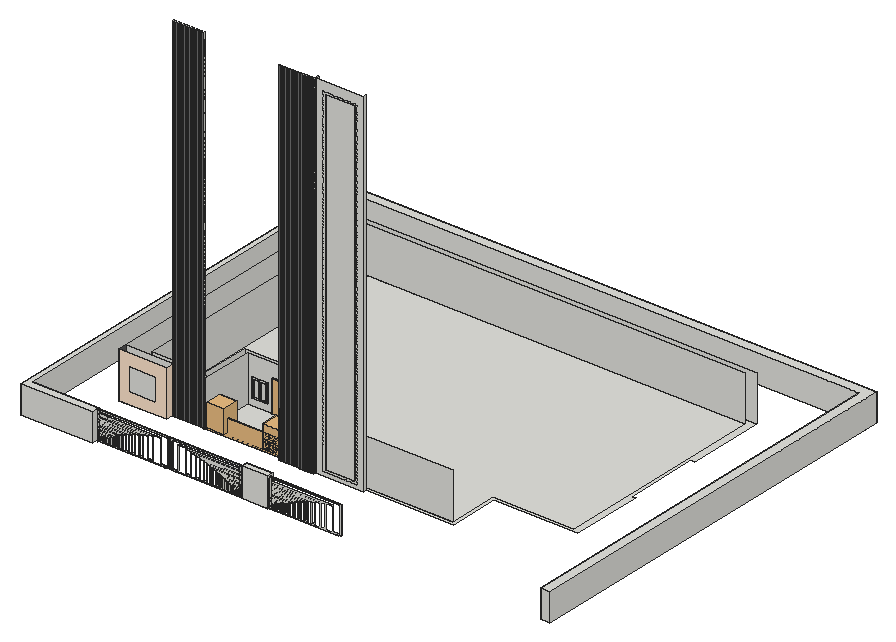
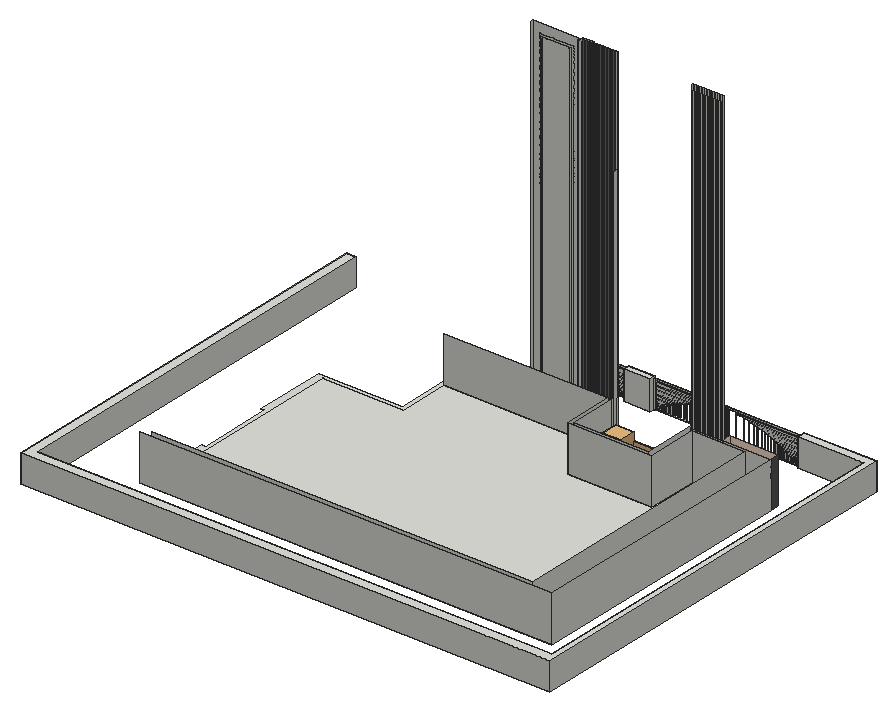
# SketchUp Ruby script. Lengths in inches.
U = 1.inch
M = Sketchup.active_model
def pt(a) = Geom::Point3d.new(a.map { |v| v * U })
def face(e, loops, mat)
  f = e.add_face(loops[0].map { |a| pt(a) })
  loops[1..].each { |l| e.add_face(l.map { |a| pt(a) }).erase! }
  f.material = f.back_material = mat if mat
  f
end
# faces: each face lists its corners as indices into pts; further lists are holes
def faces(e, pts, list, mat = nil) = list.each { |f| face(e, (f[0].is_a?(Array) ? f : [f]).map { |l| l.map { |i| pts[i] } }, mat) }
# xy, xz, yz: faces in a plane at the given z, y or x. An outline is a flat list of corners, or four numbers for a rectangle; further outlines are holes
def ring(l) = l.size == 4 ? [[l[0], l[1]], [l[2], l[1]], [l[2], l[3]], [l[0], l[3]]] : l.each_slice(2).to_a
def flat(e, list, mat, &to3) = list.each { |f| face(e, (f[0].is_a?(Array) ? f : [f]).map { |l| ring(l).map { |u, v| to3.(u, v) } }, mat) }
def xy(e, z, list, mat = nil) = flat(e, list, mat) { |x, y| [x, y, z] }
def xz(e, y, list, mat = nil) = flat(e, list, mat) { |x, z| [x, y, z] }
def yz(e, x, list, mat = nil) = flat(e, list, mat) { |y, z| [x, y, z] }
def lines(e, pts, list) = list.each { |a, b| e.add_line(pt(pts[a]), pt(pts[b])) }
# prism: a flat outline (further loops are holes) pulled along v
def prism(e, loops, v, mat = nil)
  f = face(e, loops, mat); d = Geom::Vector3d.new(v.map { |x| x * U })
  f.pushpull(f.normal.samedirection?(d) ? d.length : -d.length)
end
def box(e, o, s, mat = nil) = prism(e, [[o, [o[0] + s[0], o[1], o[2]], [o[0] + s[0], o[1] + s[1], o[2]], [o[0], o[1] + s[1], o[2]]]], [0, 0, s[2]], mat)
def at(x, y, z, deg = 0) = Geom::Transformation.translation(pt([x, y, z])) * Geom::Transformation.rotation(ORIGIN, Z_AXIS, deg.degrees)
def axes(o, x, y, z) = Geom::Transformation.new([*x, 0, *y, 0, *z, 0, *pt(o).to_a, 1])
def part(name) = M.definitions.add(name)
# library, detail: a bought-in or finely detailed component or shape, given as its bounding box
def library(name, o, s) = part(name).tap { |d| box(d.entities, o, s) }
def detail(e, o, s) = box(e.add_group.entities, o, s)
def put(e, d, t, mat = nil) = e.add_instance(d, t).tap { |i| i.material = mat if mat }
def group(e, t, mat = nil) = e.add_group.tap { |g| g.transformation = t; g.material = mat if mat }.entities
root = M.entities
M.materials.add("[Color C01]").color = [255, 229, 204]
M.materials.add("[Color M05]").color = [114, 114, 114]
M.materials.add("[Color M06]").color = [86, 86, 86]
c1 = part("Glass Door - Open Shower")
box(c1.entities,[0,0,0.95],[40,1.5,72])
c2 = library("Glass balustrade section",[0,0,0],[60.75,3.875,44.35])
c3 = library("KentiaPalm",[-22.86,-14.31,0],[47.49,43.96,59.125])
c4 = library("porta 4",[0.2,-5.42,1.33],[46.55,4.72,83.21])
c5 = part("Window")
xy(c5.entities,31.72,[[-0.78,88.6,2.72,128.1]])
xy(c5.entities,34.95,[[-0.78,91.53,0.84,106.59],[0.84,91.53,1.05,97.58],[1.05,91.53,1.42,106.59],[1.42,91.53,2.72,106.59],[0.84,97.58,1.05,98.18],
  [0.84,98.18,1.05,106.59]])
xy(c5.entities,35.27,[[-0.78,110.09,0.97,125.14],[1.05,110.09,2.72,125.14]])
xy(c5.entities,58.35,[[2.72,108.74,3.8,109.74]])
xy(c5.entities,77.8125,[[-0.78,110.09,2.72,125.14],[0.97,110.09,1.05,125.14]])
xy(c5.entities,77.93,[[-0.78,91.53,0.84,106.59],[1.05,91.53,1.42,106.59],[1.42,91.53,2.72,106.59]])
xy(c5.entities,80.72,[[-0.78,88.6,2.72,128.1]])
xz(c5.entities,88.6,[[-0.78,31.72,2.72,80.72]])
xz(c5.entities,91.53,[[-0.78,34.95,0.84,77.93],[1.05,34.95,1.42,77.93],[1.42,34.95,2.72,77.93]])
xz(c5.entities,106.59,[[-0.78,34.95,0.84,77.93],[0.84,34.95,1.05,77.93],[0.84,34.95,2.72,77.93]])
xz(c5.entities,108.74,[[3.8,54.35,4.22,54.6,4.22,59.47,2.72,59.97,2.72,58.35,3.8,58.35]])
xz(c5.entities,109.74,[[3.8,54.35,3.8,58.35,2.72,58.35,2.72,59.97,4.22,59.47,4.22,54.6]])
xz(c5.entities,110.09,[[-0.78,35.27,0.97,77.8125],[1.05,35.27,2.72,77.8125]])
xz(c5.entities,125.14,[[-0.78,35.27,0.97,77.8125],[0.97,35.27,1.05,80.72],[1.05,35.27,2.72,77.8125]])
xz(c5.entities,128.1,[[-0.78,31.72,2.72,80.72]])
yz(c5.entities,-0.78,[[[88.6,31.72,128.1,80.72],[91.53,34.95,106.59,77.93],[110.09,35.27,125.14,77.8125]]])
yz(c5.entities,0.84,[[91.53,34.95,106.59,77.93]])
yz(c5.entities,0.97,[[110.09,35.27,125.14,77.8125]])
yz(c5.entities,1.05,[[91.53,34.95,106.59,77.93],[110.09,35.27,125.14,77.8125]])
yz(c5.entities,1.42,[[91.53,34.95,106.59,77.93]])
yz(c5.entities,2.72,[[[88.6,31.72,108.35,80.72],[91.53,34.95,106.59,77.93]],[[108.35,31.72,128.1,80.72],[110.09,35.27,125.14,77.8125],[108.74,58.35,109.74,59.97]]])
yz(c5.entities,3.8,[[108.74,54.35,109.74,58.35]])
yz(c5.entities,4.22,[[108.74,54.6,109.74,59.47]])
p = [[4.22,108.74,54.6],[3.8,108.74,54.35],[3.8,109.74,54.35],[4.22,109.74,54.6],[2.72,109.74,59.97],[2.72,108.74,59.97],
  [4.22,108.74,59.47],[4.22,109.74,59.47],[-0.78,86.4,89.94],[-0.78,86.44,89.94],[15.22,130.69,89.94],[15.22,130.65,89.94],
  [-0.78,86.44,28.19],[-0.78,86.4,28.19],[7.72,130.69,89.94],[7.72,130.65,89.94]]
faces(c5.entities,p,[[0,1,2,3],[4,5,6,7]])
lines(c5.entities,p,[[8,9],[10,11],[12,13],[14,15]])
box(root,[569.26,11.31,0],[68.62,15.69,75.8125])
prism(root,[[[0,1064.875,0],[1383.3125,1064.875,0],[1383.3125,0,0],[1358.82,0,0],[1358.82,1038.875,0],[15.91,1038.875,0],[15.91,21.72,0],[188.09,21.72,0],[188.09,0,0],[0,0,0]]],[0,0,72.6875])
xy(root,0,[[528.5625,182.3125,534.875,184.75],[535.75,182.3125,542.0625,184.75],[542.5,182.3125,548.8125,184.75],[549.375,182.3125,555.6875,184.75],[556.1875,182.3125,562.5,184.75],
  [563.1875,182.3125,569.5,184.75],[570.1875,182.3125,576.5,184.75],[577,182.3125,583.3125,184.75],[584.75,182.3125,591.0625,184.75],[592,182.3125,598.3125,184.75],
  [599.375,182.3125,605.6875,184.75],[606.75,182.3125,613.07,184.75],[614.13,182.3125,620.44,184.75],[[528.67,184.75,620.44,184.75,620.44,195.5625,622.95,195.5625,622.95,187.0625,747.02,187.0625,747.02,195.5625,974.8125,195.5625,974.8125,325.5625,1196,325.5625,1196,513.49,1186.5,513.49,1186.5,706.47,1196,706.47,1196,908.0625,119.8125,908.0625,119.8125,195.5625,327.85,195.5625,327.85,189.875,333.1,189.875,333.1,325.5625,528.67,325.5625],[180.5,204.5625,180.5,894.25,1177.5,894.25,1177.5,334.5625,965.8125,334.5625,965.8125,204.5625,537.67,204.5625,537.67,334.5625,318.85,334.5625,318.85,204.5625]],[244.96,193.5625,325.71,195.5625],
  [333.1,195.5625,528.67,325.5625],[180.5,204.5625,318.85,204.5625,318.85,334.5625,537.67,334.5625,537.67,204.5625,965.8125,204.5625,965.8125,334.5625,1177.5,334.5625,1177.5,894.25,180.5,894.25]])
xy(root,0,[[245.08,191.125,251.39,193.5625],[251.83,191.125,258.14,193.5625],[258.52,191.125,264.83,193.5625],[265.14,191.125,271.46,193.5625],[271.89,191.125,278.21,193.5625],
  [278.64,191.125,284.96,193.5625],[285.46,191.125,291.77,193.5625],[292.21,191.125,298.52,193.5625],[299.02,191.125,305.33,193.5625],[305.83,191.125,312.14,193.5625],
  [312.71,191.125,319.02,193.5625],[319.39,191.125,325.71,193.5625]],"[Color M05]")
xy(root,0,[[119.8125,172.4375,244.96,195.5625]],"[Color M06]")
xy(root,0.49,[[193.54,13.81,370.76,14.31],[385.35,13.81,562.58,14.31],[643.44,13.81,820.67,14.31]])
xy(root,0.7,[[187.97,14.12,191.63,15.56],[372.66,14.12,376.32,15.56],[379.79,14.12,383.45,15.56],[564.48,14.12,568.14,15.56],[637.88,14.12,641.54,15.56]])
xy(root,3.2,[[197.6875,13.81,203.4375,14.31],[206.84,13.81,212.06,14.31],[216.11,13.81,221.45,14.31],[226.23,13.81,231.97,14.31],[237.375,13.81,243.66,14.31],
  [249.79,13.81,256.71,14.31],[263.81,13.81,271.47,14.31],[279.92,13.81,288.49,14.31],[298.9,13.81,308.95,14.31],[321.26,13.81,335.28,14.31],
  [354.73,13.81,366.2,14.31],[366.2,13.81,370.76,14.31],[385.35,13.81,389.91,14.31],[389.91,13.81,401.38,14.31],[420.83,13.81,434.85,14.31],
  [447.17,13.81,457.21,14.31],[467.62,13.81,476.19,14.31],[484.64,13.81,492.31,14.31],[499.4,13.81,506.32,14.31],[512.45,13.81,518.74,14.31],
  [524.14,13.81,529.88,14.31],[534.66,13.81,540,14.31],[544.05,13.81,549.28,14.31],[552.68,13.81,558.43,14.31],[647.59,13.81,653.34,14.31],
  [656.74,13.81,661.97,14.31],[666.01,13.81,671.36,14.31],[676.14,13.81,681.88,14.31],[687.28,13.81,693.57,14.31],[699.7,13.81,706.61,14.31],
  [713.71,13.81,721.38,14.31],[729.83,13.81,738.4,14.31],[748.81,13.81,758.85,14.31]])
xy(root,3.7,[[475.4,13.73,468.41,13.8,468.41,14.31,475.4,14.31],[730.62,13.73,737.61,13.8,737.61,14.31,730.62,14.31],[299.6875,13.93,308.16,14.02,308.16,14.31,299.6875,14.31],[456.42,13.93,447.95,14.02,447.95,14.31,456.42,14.31],[749.6,13.93,758.07,14.02,758.07,14.31,749.6,14.31],
  [322.05,14.17,334.49,14.31,322.05,14.31],[434.07,14.17,421.62,14.31,434.07,14.31]])
xy(root,5.63,[[196.38,13.81,200.95,14.31],[555.16,13.81,559.73,14.31],[646.29,13.81,650.86,14.31]])
xy(root,6.62,[[193.54,13.81,194.89,14.31],[194.89,13.81,196.01,14.31],[196.01,13.81,203.4375,14.31],[552.68,13.81,560.1,14.31],[560.1,13.81,561.22,14.31],
  [561.22,13.81,562.58,14.31],[643.44,13.81,644.8,14.31],[644.8,13.81,645.92,14.31],[645.92,13.81,653.34,14.31]])
xy(root,9.32,[[193.54,13.81,199.38,14.31],[199.38,13.81,200.99,14.31],[200.99,13.81,206.84,14.31],[549.28,13.81,555.12,14.31],[555.12,13.81,556.73,14.31],
  [556.73,13.81,562.58,14.31],[643.44,13.81,649.29,14.31],[649.29,13.81,650.9,14.31],[650.9,13.81,656.74,14.31]])
xy(root,12.74,[[193.54,13.81,204.26,14.31],[204.26,13.81,212.06,14.31],[544.05,13.81,551.85,14.31],[551.85,13.81,562.58,14.31],[643.44,13.81,654.17,14.31],
  [654.17,13.81,661.97,14.31]])
xy(root,15.44,[[193.54,13.81,209.89,14.31],[209.89,13.81,216.11,14.31],[540,13.81,546.22,14.31],[546.22,13.81,562.58,14.31],[643.44,13.81,659.79,14.31],
  [659.79,13.81,666.01,14.31]])
xy(root,17.65,[[647.73,187.0625,723.37,190.9375]])
xy(root,18.86,[[193.54,13.81,213.58,14.31],[213.58,13.81,221.45,14.31],[534.66,13.81,542.53,14.31],[542.53,13.81,562.58,14.31],[643.44,13.81,663.48,14.31],
  [663.48,13.81,671.36,14.31]])
xy(root,21.57,[[193.54,13.81,219.5625,14.31],[219.5625,13.81,226.23,14.31],[529.88,13.81,536.55,14.31],[536.55,13.81,562.58,14.31],[643.44,13.81,669.47,14.31],
  [669.47,13.81,676.14,14.31]])
xy(root,24.98,[[193.54,13.81,223.73,14.31],[223.73,13.81,231.97,14.31],[524.14,13.81,532.38,14.31],[532.38,13.81,562.58,14.31],[643.44,13.81,673.64,14.31],
  [673.64,13.81,681.88,14.31]])
xz(root,14.12,[[187.97,0.7,187.97,73.2,376.32,73.2,376.32,0.7,372.66,0.7,372.66,70.9,191.63,70.9,191.63,0.7],[379.79,0.7,383.45,0.7,383.45,70.9,564.48,70.9,564.48,0.7,568.14,0.7,568.14,73.2,379.79,73.2],[637.88,0.7,637.88,73.2,826.23,73.2,826.23,0.7,822.57,0.7,822.57,70.9,641.54,70.9,641.54,0.7]])
xz(root,14.31,[[[192.75,0,192.75,3.7,196.01,6.12,202.65,6.12,199.38,3.7,202.65,3.7,202.65,6.12,192.75,6.12,192.75,9.82,207.625,9.82,207.625,3.7,211.27,3.7,211.27,12.24,192.75,12.24,192.75,15.9375,216.9,15.9375,216.9,3.7,220.67,3.7,220.67,18.36,192.75,18.36,192.75,22.06,227.02,22.06,227.02,3.7,231.18,3.7,231.18,24.48,192.75,24.48,192.75,28.18,238.16,28.18,238.16,3.7,242.875,3.7,242.875,30.61,192.75,30.61,192.75,34.3,250.58,34.3,250.58,3.7,255.92,3.7,255.92,36.73,192.75,36.73,192.75,40.42,264.59,40.42,264.59,3.7,270.68,3.7,270.68,42.85,192.75,42.85,192.75,46.54,280.71,46.54,280.71,3.7,287.71,3.7,287.71,48.97,192.75,48.97,192.75,52.67,299.6875,52.67,299.6875,3.7,308.16,3.7,308.16,55.09,192.75,55.09,192.75,58.79,322.05,58.79,322.05,3.7,334.49,3.7,334.49,61.21,192.75,61.21,192.75,64.91,355.52,64.91,355.52,3.7,371.55,3.7,371.55,0],[193.54,0.49,370.76,0.49,370.76,3.2,354.73,3.2,354.73,64.41,193.54,64.41,193.54,61.71,335.28,61.71,335.28,3.2,321.26,3.2,321.26,58.29,193.54,58.29,193.54,55.59,308.95,55.59,308.95,3.2,298.9,3.2,298.9,52.17,193.54,52.17,193.54,49.46,288.49,49.46,288.49,3.2,279.92,3.2,279.92,46.05,193.54,46.05,193.54,43.34,271.47,43.34,271.47,3.2,263.81,3.2,263.81,39.93,193.54,39.93,193.54,37.22,256.71,37.22,256.71,3.2,249.79,3.2,249.79,33.81,193.54,33.81,193.54,31.1,243.66,31.1,243.66,3.2,237.375,3.2,237.375,27.6875,193.54,27.6875,193.54,24.98,231.97,24.98,231.97,3.2,226.23,3.2,226.23,21.57,193.54,21.57,193.54,18.86,221.45,18.86,221.45,3.2,216.11,3.2,216.11,15.44,193.54,15.44,193.54,12.74,212.06,12.74,212.06,3.2,206.84,3.2,206.84,9.32,193.54,9.32,193.54,6.62,203.4375,6.62,203.4375,3.2,197.6875,3.2,200.95,5.63,196.38,5.63,193.54,3.52]],[[384.5625,0,563.36,0,563.36,3.7,560.1,6.12,553.46,6.12,556.73,3.7,553.46,3.7,553.46,6.12,563.36,6.12,563.36,9.82,548.49,9.82,548.49,3.7,544.84,3.7,544.84,12.24,563.36,12.24,563.36,15.9375,539.22,15.9375,539.22,3.7,535.45,3.7,535.45,18.36,563.36,18.36,563.36,22.06,529.09,22.06,529.09,3.7,524.93,3.7,524.93,24.48,563.36,24.48,563.36,28.18,517.95,28.18,517.95,3.7,513.24,3.7,513.24,30.61,563.36,30.61,563.36,34.3,505.53,34.3,505.53,3.7,500.19,3.7,500.19,36.73,563.36,36.73,563.36,40.42,491.52,40.42,491.52,3.7,485.43,3.7,485.43,42.85,563.36,42.85,563.36,46.54,475.4,46.54,475.4,3.7,468.41,3.7,468.41,48.97,563.36,48.97,563.36,52.67,456.42,52.67,456.42,3.7,447.95,3.7,447.95,55.09,563.36,55.09,563.36,58.79,434.07,58.79,434.07,3.7,421.62,3.7,421.62,61.21,563.36,61.21,563.36,64.91,400.59,64.91,400.59,3.7,384.5625,3.7],[385.35,0.49,385.35,3.2,401.38,3.2,401.38,64.41,562.58,64.41,562.58,61.71,420.83,61.71,420.83,3.2,434.85,3.2,434.85,58.29,562.58,58.29,562.58,55.59,447.17,55.59,447.17,3.2,457.21,3.2,457.21,52.17,562.58,52.17,562.58,49.46,467.62,49.46,467.62,3.2,476.19,3.2,476.19,46.05,562.58,46.05,562.58,43.34,484.64,43.34,484.64,3.2,492.31,3.2,492.31,39.93,562.58,39.93,562.58,37.22,499.4,37.22,499.4,3.2,506.32,3.2,506.32,33.81,562.58,33.81,562.58,31.1,512.45,31.1,512.45,3.2,518.74,3.2,518.74,27.6875,562.58,27.6875,562.58,24.98,524.14,24.98,524.14,3.2,529.88,3.2,529.88,21.57,562.58,21.57,562.58,18.86,534.66,18.86,534.66,3.2,540,3.2,540,15.44,562.58,15.44,562.58,12.74,544.05,12.74,544.05,3.2,549.28,3.2,549.28,9.32,562.58,9.32,562.58,6.62,552.68,6.62,552.68,3.2,558.43,3.2,555.16,5.63,559.73,5.63,562.58,3.52,562.58,0.49]],[[642.65,0,642.65,3.7,645.92,6.12,652.55,6.12,649.29,3.7,652.55,3.7,652.55,6.12,642.65,6.12,642.65,9.82,657.53,9.82,657.53,3.7,661.18,3.7,661.18,12.24,642.65,12.24,642.65,15.9375,666.8,15.9375,666.8,3.7,670.57,3.7,670.57,18.36,642.65,18.36,642.65,22.06,676.92,22.06,676.92,3.7,681.09,3.7,681.09,24.48,642.65,24.48,642.65,28.18,688.07,28.18,688.07,3.7,692.78,3.7,692.78,30.61,642.65,30.61,642.65,34.3,700.48,34.3,700.48,3.7,705.83,3.7,705.83,36.73,642.65,36.73,642.65,40.42,714.5,40.42,714.5,3.7,720.59,3.7,720.59,42.85,642.65,42.85,642.65,46.54,730.62,46.54,730.62,3.7,737.61,3.7,737.61,48.97,642.65,48.97,642.65,52.67,749.6,52.67,749.6,3.7,758.07,3.7,758.07,55.09,642.65,55.09,642.65,58.79,771.95,58.79,771.95,3.7,784.4,3.7,784.4,61.21,642.65,61.21,642.65,64.91,805.43,64.91,805.43,3.7,821.45,3.7,821.45,0],[643.44,0.49,820.67,0.49,820.67,3.2,804.64,3.2,804.64,64.41,643.44,64.41,643.44,61.71,785.19,61.71,785.19,3.2,771.16,3.2,771.16,58.29,643.44,58.29,643.44,55.59,758.85,55.59,758.85,3.2,748.81,3.2,748.81,52.17,643.44,52.17,643.44,49.46,738.4,49.46,738.4,3.2,729.83,3.2,729.83,46.05,643.44,46.05,643.44,43.34,721.38,43.34,721.38,3.2,713.71,3.2,713.71,39.93,643.44,39.93,643.44,37.22,706.61,37.22,706.61,3.2,699.7,3.2,699.7,33.81,643.44,33.81,643.44,31.1,693.57,31.1,693.57,3.2,687.28,3.2,687.28,27.6875,643.44,27.6875,643.44,24.98,681.88,24.98,681.88,3.2,676.14,3.2,676.14,21.57,643.44,21.57,643.44,18.86,671.36,18.86,671.36,3.2,666.01,3.2,666.01,15.44,643.44,15.44,643.44,12.74,661.97,12.74,661.97,3.2,656.74,3.2,656.74,9.32,643.44,9.32,643.44,6.62,653.34,6.62,653.34,3.2,647.59,3.2,650.86,5.63,646.29,5.63,643.44,3.52]],[200.99,9.82,204.18,12.18,204.26,12.24,211.27,12.24,207.95,10.06,207.625,9.82],[548.49,9.82,555.12,9.82,551.9375,12.18,551.85,12.24,544.84,12.24,548.16,10.06],
  [650.9,9.82,654.08,12.18,654.17,12.24,661.18,12.24,657.85,10.06,657.53,9.82],[209.89,15.9375,213.58,18.36,220.67,18.36,219.96,17.95,216.9,15.9375],[539.22,15.9375,546.22,15.9375,542.53,18.36,535.45,18.36,536.15,17.95],[659.79,15.9375,663.48,18.36,670.57,18.36,669.87,17.95,666.8,15.9375],[219.5625,22.06,223.73,24.48,231.18,24.48,227.02,22.06],
  [529.09,22.06,536.55,22.06,532.38,24.48,524.93,24.48],[669.47,22.06,673.64,24.48,681.09,24.48,676.92,22.06]])
xz(root,14.43,[[182.38,9.21,186.86,10.5],[569.26,9.21,573.73,10.5],[632.29,9.21,636.76,10.5],[182.38,11.42,186.86,12.71],[569.26,11.42,573.73,12.71],
  [632.29,11.42,636.76,12.71]])
xz(root,15.56,[[[186.86,0,186.86,73.9,377.4375,73.9,377.4375,0,371.55,0,371.55,70.2,192.75,70.2,192.75,0],[187.97,0.7,191.63,0.7,191.63,70.9,372.66,70.9,372.66,0.7,376.32,0.7,376.32,73.2,187.97,73.2]],[[378.67,0,384.5625,0,384.5625,70.2,563.36,70.2,563.36,0,569.26,0,569.26,73.9,378.67,73.9],[379.79,0.7,379.79,73.2,568.14,73.2,568.14,0.7,564.48,0.7,564.48,70.9,383.45,70.9,383.45,0.7]],[[636.76,0,636.76,73.9,827.35,73.9,827.35,0,821.45,0,821.45,70.2,642.65,70.2,642.65,0],[637.88,0.7,641.54,0.7,641.54,70.9,822.57,70.9,822.57,0.7,826.23,0.7,826.23,73.2,637.88,73.2]]])
xz(root,172.4375,[[[119.8125,0,244.96,120],[145.1,29.54,217.17,90.15]]],"[Color C01]")
xz(root,182.3125,[[528.5625,0,534.875,924],[535.75,0,542.0625,924],[542.5,0,548.8125,924],[549.375,0,555.6875,924],[556.1875,0,562.5,924],
  [563.1875,0,569.5,924],[570.1875,0,576.5,924],[577,0,583.3125,924],[584.75,0,591.0625,924],[592,0,598.3125,924],
  [599.375,0,605.6875,924],[606.75,0,613.07,924],[614.13,0,620.44,924]],"[Color M05]")
xz(root,184.75,[[528.67,0,534.875,924],[534.875,0,535.75,924],[542.0625,0,542.5,924],[548.8125,0,549.375,924],[555.6875,0,556.1875,924],
  [562.5,0,563.1875,924],[569.5,0,570.1875,924],[576.5,0,577,924],[583.3125,0,584.75,924],[591.0625,0,592,924],
  [598.3125,0,599.375,924],[605.6875,0,606.75,924],[613.07,0,614.13,924]])
xz(root,184.75,[[535.75,0,542.0625,924],[542.5,0,548.8125,924],[549.375,0,555.6875,924],[556.1875,0,562.5,924],[563.1875,0,569.5,924],
  [570.1875,0,576.5,924],[577,0,583.3125,924],[584.75,0,591.0625,924],[592,0,598.3125,924],[599.375,0,605.6875,924],
  [606.75,0,613.07,924],[614.13,0,620.44,924]],"[Color M05]")
xz(root,187.0625,[[[622.95,0,747.02,924],[641.05,10.96,730.05,900.15]],[[641.05,10.96,730.05,900.15],[647.73,17.65,723.37,893.47]]])
xz(root,189.875,[[327.85,0,333.1,120]])
xz(root,191.125,[[245.08,0,251.39,924],[251.83,0,258.14,924],[258.52,0,264.83,924],[265.14,0,271.46,924],[271.89,0,278.21,924],
  [278.64,0,284.96,924],[285.46,0,291.77,924],[292.21,0,298.52,924],[299.02,0,305.33,924],[305.83,0,312.14,924],
  [312.71,0,319.02,924],[319.39,0,325.71,924]],"[Color M05]")
xz(root,193.5625,[[244.96,0,245.08,912],[245.08,0,251.39,912],[251.39,0,251.83,912],[251.83,0,258.14,912],[258.14,0,258.52,912],
  [258.52,0,264.83,912],[264.83,0,265.14,912],[265.14,0,271.46,912],[271.46,0,271.89,912],[271.89,0,278.21,912],
  [278.21,0,278.64,912],[278.64,0,284.96,912],[284.96,0,285.46,912],[285.46,0,291.77,912],[291.77,0,292.21,912],
  [292.21,0,298.52,912],[298.52,0,299.02,912],[299.02,0,305.33,912],[305.33,0,305.83,912],[305.83,0,312.14,912],
  [312.14,0,312.71,912],[312.71,0,319.02,912],[319.02,0,319.39,912],[319.39,0,325.71,912]])
xz(root,195.5625,[[119.8125,0,244.96,120],[244.96,0,325.71,120],[325.71,0,327.85,120],[620.44,0,622.95,120]])
xz(root,204.5625,[[180.5,0,318.85,120],[537.67,0,965.8125,120]])
xz(root,325.5625,[[333.1,0,528.67,120]])
xz(root,334.5625,[[318.85,0,537.67,120]])
xz(root,894.25,[[180.5,0,1177.5,120]])
xz(root,908.0625,[[119.8125,0,1196,120]])
yz(root,119.8125,[[195.5625,0,908.0625,120]])
yz(root,119.8125,[[172.4375,0,195.5625,120]],"[Color M06]")
yz(root,180.5,[[204.5625,0,894.25,120]])
yz(root,187.97,[[14.12,0.7,15.56,73.2]])
yz(root,191.63,[[14.12,0.7,15.56,3.7],[14.12,3.7,15.56,6.12],[14.12,6.12,15.56,9.82],[14.12,9.82,15.56,12.24],[14.12,12.24,15.56,15.9375],
  [14.12,15.9375,15.56,18.36],[14.12,18.36,15.56,22.06],[14.12,22.06,15.56,24.48],[14.12,24.48,15.56,28.18]])
yz(root,192.75,[[11.31,0,12.93,0,12.93,3.7,15.56,3.7,15.56,6.12,12.93,6.12,12.93,9.82,15.56,9.82,15.56,12.24,12.93,12.24,12.93,15.9375,15.56,15.9375,15.56,18.36,12.93,18.36,12.93,22.06,15.56,22.06,15.56,24.48,12.93,24.48,12.93,28.18,15.56,28.18,15.56,30.61,12.93,30.61,12.93,34.3,15.56,34.3,15.56,36.73,12.93,36.73,12.93,40.42,15.56,40.42,15.56,42.85,12.93,42.85,12.93,46.54,15.56,46.54,15.56,48.97,12.93,48.97,12.93,52.67,15.56,52.67,15.56,55.09,12.93,55.09,12.93,58.79,15.56,58.79,15.56,61.21,12.93,61.21,12.93,64.91,15.56,64.91,15.56,70.2,11.31,70.2],[14.31,0,15.56,3.7],[14.31,6.12,15.56,9.82],[14.31,12.24,15.56,15.9375],[14.31,18.36,15.56,22.06],
  [14.31,24.48,15.56,28.18]])
yz(root,193.54,[[13.81,0.49,14.31,3.52],[13.81,6.62,14.31,9.32],[13.81,12.74,14.31,15.44],[13.81,18.86,14.31,21.57],[13.81,24.98,14.31,27.6875]])
yz(root,203.4375,[[13.81,3.2,14.31,6.62]])
yz(root,206.84,[[13.81,3.2,14.31,9.32]])
yz(root,212.06,[[13.81,3.2,14.31,12.74]])
yz(root,216.11,[[13.81,3.2,14.31,15.44]])
yz(root,221.45,[[13.81,3.2,14.31,18.86]])
yz(root,226.23,[[13.81,3.2,14.31,21.57]])
yz(root,231.97,[[13.81,3.2,14.31,24.98]])
yz(root,237.375,[[13.81,3.2,14.31,27.6875]])
yz(root,243.66,[[13.81,3.2,14.31,31.1]])
yz(root,244.96,[[193.5625,0,195.5625,120]])
yz(root,244.96,[[172.4375,0,193.5625,120]],"[Color C01]")
yz(root,245.08,[[191.125,0,193.5625,924]])
yz(root,249.79,[[13.81,3.2,14.31,33.81]])
yz(root,251.39,[[191.125,0,193.5625,924]])
yz(root,251.83,[[191.125,0,193.5625,924]])
yz(root,256.71,[[13.81,3.2,14.31,37.22]])
yz(root,258.14,[[191.125,0,193.5625,924]])
yz(root,258.52,[[191.125,0,193.5625,924]])
yz(root,263.81,[[13.81,3.2,14.31,39.93]])
yz(root,264.83,[[191.125,0,193.5625,924]])
yz(root,265.14,[[191.125,0,193.5625,924]])
yz(root,271.46,[[191.125,0,193.5625,924]])
yz(root,271.47,[[13.81,3.2,14.31,43.34]])
yz(root,271.89,[[191.125,0,193.5625,924]])
yz(root,278.21,[[191.125,0,193.5625,924]])
yz(root,278.64,[[191.125,0,193.5625,924]])
yz(root,279.92,[[13.81,3.2,14.31,46.05]])
yz(root,284.96,[[191.125,0,193.5625,924]])
yz(root,285.46,[[191.125,0,193.5625,924]])
yz(root,288.49,[[13.81,3.2,14.31,49.46]])
yz(root,291.77,[[191.125,0,193.5625,924]])
yz(root,292.21,[[191.125,0,193.5625,924]])
yz(root,298.52,[[191.125,0,193.5625,924]])
yz(root,298.9,[[13.81,3.2,14.31,52.17]])
yz(root,299.02,[[191.125,0,193.5625,924]])
yz(root,305.33,[[191.125,0,193.5625,924]])
yz(root,305.83,[[191.125,0,193.5625,924]])
yz(root,308.95,[[13.81,3.2,14.31,55.59]])
yz(root,312.14,[[191.125,0,193.5625,924]])
yz(root,312.71,[[191.125,0,193.5625,924]])
yz(root,318.85,[[204.5625,0,334.5625,120]])
yz(root,319.02,[[191.125,0,193.5625,924]])
yz(root,319.39,[[191.125,0,193.5625,924]])
yz(root,321.26,[[13.81,3.2,14.31,58.29]])
yz(root,325.71,[[191.125,0,193.5625,924],[193.5625,0,195.5625,912]])
yz(root,327.85,[[189.875,0,195.5625,120]])
yz(root,333.1,[[189.875,0,325.5625,120]])
yz(root,335.28,[[13.81,3.2,14.31,61.71]])
yz(root,354.73,[[13.81,3.2,14.31,64.41]])
yz(root,370.76,[[13.81,0.49,14.31,3.2]])
yz(root,371.55,[[14.31,0,15.56,3.7]])
yz(root,372.66,[[14.12,0.7,15.56,3.7],[14.12,3.7,15.56,66.96]])
yz(root,376.32,[[14.12,0.7,15.56,73.2]])
yz(root,379.79,[[14.12,0.7,15.56,73.2]])
yz(root,383.45,[[14.12,0.7,15.56,3.7],[14.12,3.7,15.56,66.96]])
yz(root,384.5625,[[14.31,0,15.56,3.7]])
yz(root,385.35,[[13.81,0.49,14.31,3.2]])
yz(root,401.38,[[13.81,3.2,14.31,64.41]])
yz(root,420.83,[[13.81,3.2,14.31,61.71]])
yz(root,434.85,[[13.81,3.2,14.31,58.29]])
yz(root,447.17,[[13.81,3.2,14.31,55.59]])
yz(root,457.21,[[13.81,3.2,14.31,52.17]])
yz(root,467.62,[[13.81,3.2,14.31,49.46]])
yz(root,476.19,[[13.81,3.2,14.31,46.05]])
yz(root,484.64,[[13.81,3.2,14.31,43.34]])
yz(root,492.31,[[13.81,3.2,14.31,39.93]])
yz(root,499.4,[[13.81,3.2,14.31,37.22]])
yz(root,506.32,[[13.81,3.2,14.31,33.81]])
yz(root,512.45,[[13.81,3.2,14.31,31.1]])
yz(root,518.74,[[13.81,3.2,14.31,27.6875]])
yz(root,524.14,[[13.81,3.2,14.31,24.98]])
yz(root,528.5625,[[182.3125,0,184.75,120]])
yz(root,528.67,[[184.75,0,195.5625,648],[195.5625,0,204.5625,120],[204.5625,0,325.5625,120]])
yz(root,529.88,[[13.81,3.2,14.31,21.57]])
yz(root,534.66,[[13.81,3.2,14.31,18.86]])
yz(root,534.875,[[182.3125,0,184.75,924]])
yz(root,535.75,[[182.3125,0,184.75,924]])
yz(root,537.67,[[204.5625,0,334.5625,120]])
yz(root,540,[[13.81,3.2,14.31,15.44]])
yz(root,542.0625,[[182.3125,0,184.75,924]])
yz(root,542.5,[[182.3125,0,184.75,924]])
yz(root,544.05,[[13.81,3.2,14.31,12.74]])
yz(root,548.8125,[[182.3125,0,184.75,924]])
yz(root,549.28,[[13.81,3.2,14.31,9.32]])
yz(root,549.375,[[182.3125,0,184.75,924]])
yz(root,552.68,[[13.81,3.2,14.31,6.62]])
yz(root,555.6875,[[182.3125,0,184.75,924]])
yz(root,556.1875,[[182.3125,0,184.75,924]])
yz(root,562.5,[[182.3125,0,184.75,924]])
yz(root,562.58,[[13.81,0.49,14.31,3.52],[13.81,6.62,14.31,9.32],[13.81,12.74,14.31,15.44],[13.81,18.86,14.31,21.57],[13.81,24.98,14.31,27.6875]])
yz(root,563.1875,[[182.3125,0,184.75,924]])
yz(root,563.36,[[11.31,0,12.93,0,12.93,3.7,15.56,3.7,15.56,6.12,12.93,6.12,12.93,9.82,15.56,9.82,15.56,12.24,12.93,12.24,12.93,15.9375,15.56,15.9375,15.56,18.36,12.93,18.36,12.93,22.06,15.56,22.06,15.56,24.48,12.93,24.48,12.93,28.18,15.56,28.18,15.56,30.61,12.93,30.61,12.93,34.3,15.56,34.3,15.56,36.73,12.93,36.73,12.93,40.42,15.56,40.42,15.56,42.85,12.93,42.85,12.93,46.54,15.56,46.54,15.56,48.97,12.93,48.97,12.93,52.67,15.56,52.67,15.56,55.09,12.93,55.09,12.93,58.79,15.56,58.79,15.56,61.21,12.93,61.21,12.93,64.91,15.56,64.91,15.56,70.2,11.31,70.2],[14.31,0,15.56,3.7],[14.31,6.12,15.56,9.82],[14.31,12.24,15.56,15.9375],[14.31,18.36,15.56,22.06],
  [14.31,24.48,15.56,28.18]])
yz(root,564.48,[[14.12,0.7,15.56,3.7],[14.12,3.7,15.56,6.12],[14.12,6.12,15.56,9.82],[14.12,9.82,15.56,12.24],[14.12,12.24,15.56,15.9375],
  [14.12,15.9375,15.56,18.36],[14.12,18.36,15.56,22.06],[14.12,22.06,15.56,24.48],[14.12,24.48,15.56,28.18]])
yz(root,568.14,[[14.12,0.7,15.56,73.2]])
yz(root,569.5,[[182.3125,0,184.75,924]])
yz(root,570.1875,[[182.3125,0,184.75,924]])
yz(root,576.5,[[182.3125,0,184.75,924]])
yz(root,577,[[182.3125,0,184.75,924]])
yz(root,583.3125,[[182.3125,0,184.75,924]])
yz(root,584.75,[[182.3125,0,184.75,924]])
yz(root,591.0625,[[182.3125,0,184.75,924]])
yz(root,592,[[182.3125,0,184.75,924]])
yz(root,598.3125,[[182.3125,0,184.75,924]])
yz(root,599.375,[[182.3125,0,184.75,924]])
yz(root,605.6875,[[182.3125,0,184.75,924]])
yz(root,606.75,[[182.3125,0,184.75,924]])
yz(root,613.07,[[182.3125,0,184.75,924]])
yz(root,614.13,[[182.3125,0,184.75,924]])
yz(root,620.44,[[182.3125,0,184.75,924],[184.75,0,195.5625,924]])
yz(root,622.95,[[187.0625,0,195.5625,924]])
yz(root,637.88,[[14.12,0.7,15.56,73.2]])
yz(root,641.54,[[14.12,0.7,15.56,3.7],[14.12,3.7,15.56,6.12],[14.12,6.12,15.56,9.82],[14.12,9.82,15.56,12.24],[14.12,12.24,15.56,15.9375],
  [14.12,15.9375,15.56,18.36],[14.12,18.36,15.56,22.06],[14.12,22.06,15.56,24.48],[14.12,24.48,15.56,28.18]])
yz(root,642.65,[[11.31,0,12.93,0,12.93,3.7,15.56,3.7,15.56,6.12,12.93,6.12,12.93,9.82,15.56,9.82,15.56,12.24,12.93,12.24,12.93,15.9375,15.56,15.9375,15.56,18.36,12.93,18.36,12.93,22.06,15.56,22.06,15.56,24.48,12.93,24.48,12.93,28.18,15.56,28.18,15.56,30.61,12.93,30.61,12.93,34.3,15.56,34.3,15.56,36.73,12.93,36.73,12.93,40.42,15.56,40.42,15.56,42.85,12.93,42.85,12.93,46.54,15.56,46.54,15.56,48.97,12.93,48.97,12.93,52.67,15.56,52.67,15.56,55.09,12.93,55.09,12.93,58.79,15.56,58.79,15.56,61.21,12.93,61.21,12.93,64.91,15.56,64.91,15.56,70.2,11.31,70.2],[14.31,0,15.56,3.7],[14.31,6.12,15.56,9.82],[14.31,12.24,15.56,15.9375],[14.31,18.36,15.56,22.06],
  [14.31,24.48,15.56,28.18]])
yz(root,643.44,[[13.81,0.49,14.31,3.52],[13.81,6.62,14.31,9.32],[13.81,12.74,14.31,15.44],[13.81,18.86,14.31,21.57],[13.81,24.98,14.31,27.6875]])
yz(root,647.73,[[187.0625,17.65,190.9375,893.47]])
yz(root,653.34,[[13.81,3.2,14.31,6.62]])
yz(root,656.74,[[13.81,3.2,14.31,9.32]])
yz(root,661.97,[[13.81,3.2,14.31,12.74]])
yz(root,666.01,[[13.81,3.2,14.31,15.44]])
yz(root,671.36,[[13.81,3.2,14.31,18.86]])
yz(root,676.14,[[13.81,3.2,14.31,21.57]])
yz(root,681.88,[[13.81,3.2,14.31,24.98]])
yz(root,687.28,[[13.81,3.2,14.31,27.6875]])
yz(root,693.57,[[13.81,3.2,14.31,31.1]])
yz(root,699.7,[[13.81,3.2,14.31,33.81]])
yz(root,706.61,[[13.81,3.2,14.31,37.22]])
yz(root,713.71,[[13.81,3.2,14.31,39.93]])
yz(root,721.38,[[13.81,3.2,14.31,43.34]])
yz(root,723.37,[[187.0625,17.65,190.9375,893.47]])
yz(root,729.83,[[13.81,3.2,14.31,46.05]])
yz(root,738.4,[[13.81,3.2,14.31,49.46]])
yz(root,747.02,[[187.0625,0,195.5625,924]])
yz(root,748.81,[[13.81,3.2,14.31,52.17]])
p = [[200.95,14.31,5.63],[197.6875,14.31,3.2],[197.6875,13.81,3.2],[200.95,13.81,5.63],[555.16,14.31,5.63],[558.43,14.31,3.2],
  [558.43,13.81,3.2],[555.16,13.81,5.63],[650.86,14.31,5.63],[647.59,14.31,3.2],[647.59,13.81,3.2],[650.86,13.81,5.63],
  [193.54,14.31,3.52],[196.38,14.31,5.63],[196.38,13.81,5.63],[193.54,13.81,3.52],[562.58,14.31,3.52],[559.73,14.31,5.63],
  [559.73,13.81,5.63],[562.58,13.81,3.52],[643.44,14.31,3.52],[646.29,14.31,5.63],[646.29,13.81,5.63],[643.44,13.81,3.52]]
faces(root,p,[[0,1,2,3],[4,5,6,7],[8,9,10,11],[12,13,14,15],[16,17,18,19],[20,21,22,23]])
put(root,c1,axes([648.17,187.5,6.04],[1.87,0,0],[0,-0.29167,0],[0,0,12.16422]))
put(root,c2,axes([319.68,196.75,-4.5625],[3.43531,0,0],[0,1,0],[0,0,1]))
put(root,c3,at(355.95,202.91,4.82))
put(root,c3,at(498.52,211.06,1.01))
put(root,c4,at(400.125,325.5625,0.05))
put(root,c5,at(475.11,324.12,-13.16,90))
put(root,c5,at(592.54,324.12,-13.16,90))
